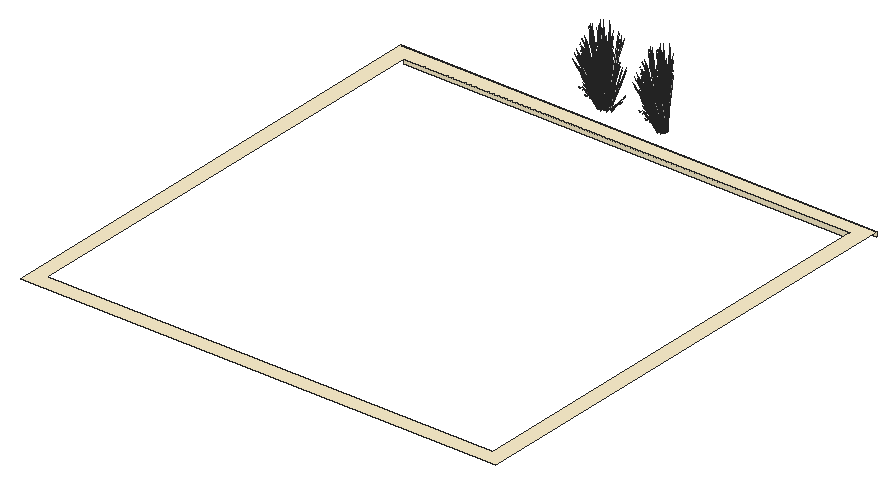
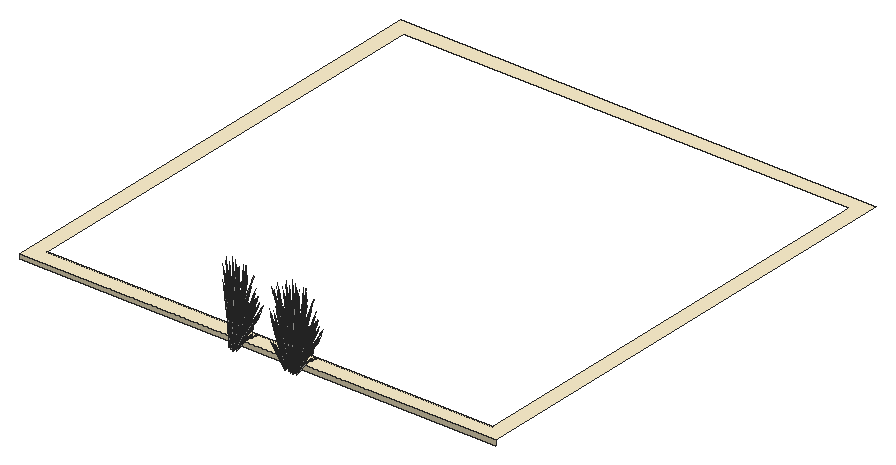
# SketchUp Ruby script. Lengths in inches.
U = 1.inch
M = Sketchup.active_model
def pt(a) = Geom::Point3d.new(a.map { |v| v * U })
def face(e, loops, mat)
  f = e.add_face(loops[0].map { |a| pt(a) })
  loops[1..].each { |l| e.add_face(l.map { |a| pt(a) }).erase! }
  f.material = f.back_material = mat if mat
  f
end
# faces: each face lists its corners as indices into pts; further lists are holes
def faces(e, pts, list, mat = nil) = list.each { |f| face(e, (f[0].is_a?(Array) ? f : [f]).map { |l| l.map { |i| pts[i] } }, mat) }
# xy, xz, yz: faces in a plane at the given z, y or x. An outline is a flat list of corners, or four numbers for a rectangle; further outlines are holes
def ring(l) = l.size == 4 ? [[l[0], l[1]], [l[2], l[1]], [l[2], l[3]], [l[0], l[3]]] : l.each_slice(2).to_a
def flat(e, list, mat, &to3) = list.each { |f| face(e, (f[0].is_a?(Array) ? f : [f]).map { |l| ring(l).map { |u, v| to3.(u, v) } }, mat) }
def xy(e, z, list, mat = nil) = flat(e, list, mat) { |x, y| [x, y, z] }
def xz(e, y, list, mat = nil) = flat(e, list, mat) { |x, z| [x, y, z] }
def yz(e, x, list, mat = nil) = flat(e, list, mat) { |y, z| [x, y, z] }
def lines(e, pts, list) = list.each { |a, b| e.add_line(pt(pts[a]), pt(pts[b])) }
# prism: a flat outline (further loops are holes) pulled along v
def prism(e, loops, v, mat = nil)
  f = face(e, loops, mat); d = Geom::Vector3d.new(v.map { |x| x * U })
  f.pushpull(f.normal.samedirection?(d) ? d.length : -d.length)
end
def box(e, o, s, mat = nil) = prism(e, [[o, [o[0] + s[0], o[1], o[2]], [o[0] + s[0], o[1] + s[1], o[2]], [o[0], o[1] + s[1], o[2]]]], [0, 0, s[2]], mat)
def at(x, y, z, deg = 0) = Geom::Transformation.translation(pt([x, y, z])) * Geom::Transformation.rotation(ORIGIN, Z_AXIS, deg.degrees)
def axes(o, x, y, z) = Geom::Transformation.new([*x, 0, *y, 0, *z, 0, *pt(o).to_a, 1])
def part(name) = M.definitions.add(name)
# library, detail: a bought-in or finely detailed component or shape, given as its bounding box
def library(name, o, s) = part(name).tap { |d| box(d.entities, o, s) }
def detail(e, o, s) = box(e.add_group.entities, o, s)
def put(e, d, t, mat = nil) = e.add_instance(d, t).tap { |i| i.material = mat if mat }
def group(e, t, mat = nil) = e.add_group.tap { |g| g.transformation = t; g.material = mat if mat }.entities
root = M.entities
M.materials.add("D01_Frost_White").color = [255, 242, 206]
M.materials.add("LightPink_Translucent").color = [144, 107, 117]
M.materials["LightPink_Translucent"].alpha = 0.75
c1 = part("blade")
p = [[2.15,0.21,22],[0,0.17,0],[0.09,0.45,0],[2.18,0.31,22],[2.29,0.31,22],[0.38,0.45,0],
  [2.48,0.24,33],[2.49,0.24,33],[2.48,0.22,33]]
faces(c1.entities,p,[[0,1,2,3],[4,5,2,3],[6,3,4,7],[8,0,3,6]])
c2 = part("seeds")
p = [[0.3,-0.1,1.38],[-0.01,-0.03,1.59],[-0.01,-0.03,0.03],[0.14,-0.07,-0.07],[0.29,-0.03,3],[0.15,0.01,3.11]]
faces(c2.entities,p,[[0,1,2,3],[1,0,4,5]],"LightPink_Translucent")
c3 = part("blade with seeds")
put(c3.entities,c1,at(0,0,0))
put(c3.entities,c2,axes([2.4,0.25,30.99],[1.5799,-0.05474,1.17369],[-0.12525,1.92788,0.29478],[-0.07173,-0.02425,1.56792]))
xy(root,2,[[[660.12,282,852,474],[666.12,288,846,468]]],"D01_Frost_White")
xz(root,468,[[666.12,0,846,2]],"D01_Frost_White")
xz(root,474,[[660.12,0,852,2]],"D01_Frost_White")
put(root,c3,axes([735.64,479.97,3.9375],[0.10505,0.10498,0.85688],[-0.48542,0.08838,0.06928],[-0.10971,-0.1648,0.36631]))
put(root,c3,axes([759.85,479.97,3.9375],[0.10505,0.10498,0.85688],[-0.48542,0.08838,0.06928],[-0.10971,-0.1648,0.36631]))
put(root,c3,axes([736.45,479.28,4.36],[-0.07029,-0.04584,0.87472],[-0.46908,0.02906,-0.13834],[-0.07486,-0.10965,0.07015]))
put(root,c3,axes([760.65,479.28,4.36],[-0.07029,-0.04584,0.87472],[-0.46908,0.02906,-0.13834],[-0.07486,-0.10965,0.07015]))
put(root,c3,axes([737.53,479.82,3.3],[-0.13063,0.06618,0.71501],[-0.39122,-0.11583,-0.15377],[0.07252,-0.14406,0.3057]))
put(root,c3,axes([761.74,479.82,3.3],[-0.13063,0.06618,0.71501],[-0.39122,-0.11583,-0.15377],[0.07252,-0.14406,0.3057]))
put(root,c3,axes([736.9375,480.05,4.49],[-0.21934,-0.26585,-0.35523],[0.45151,-0.14816,0.04287],[-0.05129,-0.12845,0.5025]))
put(root,c3,axes([761.14,480.05,4.49],[-0.21934,-0.26585,-0.35523],[0.45151,-0.14816,0.04287],[-0.05129,-0.12845,0.5025]))
put(root,c3,axes([735.51,479.69,3.3],[-0.02783,0.10696,0.71501],[-0.40683,0.08954,-0.15377],[-0.0951,-0.13825,0.3057]))
put(root,c3,axes([759.71,479.69,3.3],[-0.02783,0.10696,0.71501],[-0.40683,0.08954,-0.15377],[-0.0951,-0.13825,0.3057]))
put(root,c3,axes([736.56,479.46,2.75],[-0.07708,0.01178,0.88171],[-0.42627,-0.1326,-0.1347],[0.00715,-0.1106,0.15018]))
put(root,c3,axes([760.76,479.46,2.75],[-0.07708,0.01178,0.88171],[-0.42627,-0.1326,-0.1347],[0.00715,-0.1106,0.15018]))
put(root,c3,axes([737.85,480.31,4.49],[0.01196,-0.30243,-0.35523],[0.50354,0.02031,0.04287],[0.05314,-0.12813,0.5025]))
put(root,c3,axes([762.05,480.31,4.49],[0.01196,-0.30243,-0.35523],[0.50354,0.02031,0.04287],[0.05314,-0.12813,0.5025]))
put(root,c3,axes([738.55,479.84,4.36],[-0.00444,-0.06507,0.87472],[-0.37468,-0.18807,-0.13834],[0.05793,-0.114,0.07015]))
put(root,c3,axes([762.75,479.84,4.36],[-0.00444,-0.06507,0.87472],[-0.37468,-0.18807,-0.13834],[0.05793,-0.114,0.07015]))
put(root,c3,axes([736.98,479.82,4.26],[0.13855,-0.25143,-0.17707],[0.4042,0.07334,0.2286],[-0.03706,-0.10123,0.4374]))
put(root,c3,axes([761.18,479.82,4.26],[0.13855,-0.25143,-0.17707],[0.4042,0.07334,0.2286],[-0.03706,-0.10123,0.4374]))
put(root,c3,axes([737.28,480.16,3.9375],[-0.08557,0.11238,0.85688],[-0.35897,-0.23257,0.06928],[0.16194,-0.14495,0.36631]))
put(root,c3,axes([738.45,479.6,4.35],[-0.04667,0.02497,0.88692],[-0.45726,-0.08426,-0.08381],[-0.01655,-0.10898,0.15695]))
put(root,c3,axes([762.65,479.6,4.35],[-0.04667,0.02497,0.88692],[-0.45726,-0.08426,-0.08381],[-0.01655,-0.10898,0.15695]))
put(root,c3,axes([736.77,480,4.34],[-0.45175,-0.08196,-0.25549],[0.15485,-0.28101,-0.1979],[-0.04142,-0.11314,0.48886]))
put(root,c3,axes([760.97,480,4.34],[-0.45175,-0.08196,-0.25549],[0.15485,-0.28101,-0.1979],[-0.04142,-0.11314,0.48886]))
put(root,c3,axes([737.05,479.29,3.38],[0.05895,0.19066,0.5743],[-0.32704,-0.1056,0.42196],[0.03519,-0.09762,0.12649]))
put(root,c3,axes([761.25,479.29,3.38],[0.05895,0.19066,0.5743],[-0.32704,-0.1056,0.42196],[0.03519,-0.09762,0.12649]))
put(root,c3,axes([737.75,480.21,4.34],[-0.32898,-0.21969,-0.25549],[0.34753,-0.1924,-0.1979],[0.05006,-0.11162,0.48886]))
put(root,c3,axes([761.95,480.21,4.34],[-0.32898,-0.21969,-0.25549],[0.34753,-0.1924,-0.1979],[0.05006,-0.11162,0.48886]))
put(root,c3,axes([735.96,479.125,4.35],[-0.00857,0.03919,0.88692],[-0.42284,0.14223,-0.08381],[-0.12443,-0.0727,0.15695]))
put(root,c3,axes([760.17,479.125,4.35],[-0.00857,0.03919,0.88692],[-0.42284,0.14223,-0.08381],[-0.12443,-0.0727,0.15695]))
put(root,c3,axes([735.87,479.82,4.55],[0.51193,-0.08404,0.26881],[0.08885,0.32966,0.22165],[-0.1204,-0.09716,0.55625]))
put(root,c3,axes([760.07,479.82,4.55],[0.51193,-0.08404,0.26881],[0.08885,0.32966,0.22165],[-0.1204,-0.09716,0.55625]))
put(root,c3,axes([737.03,479.88,4.37],[0.45283,0.08548,0.24001],[-0.15485,0.28101,0.1979],[-0.02721,-0.11051,0.49665]))
put(root,c3,axes([761.23,479.88,4.37],[0.45283,0.08548,0.24001],[-0.15485,0.28101,0.1979],[-0.02721,-0.11051,0.49665]))
put(root,c3,axes([737.16,479.98,4.52],[-0.44971,0.15222,-0.0608],[-0.221,-0.27017,-0.33747],[-0.05933,-0.11385,0.51278]))
put(root,c3,axes([761.36,479.98,4.52],[-0.44971,0.15222,-0.0608],[-0.221,-0.27017,-0.33747],[-0.05933,-0.11385,0.51278]))
put(root,c3,axes([738.09,480.32,4.52],[-0.50507,-0.0162,-0.0608],[0.01381,-0.30672,-0.33747],[0.03508,-0.11813,0.51278]))
put(root,c3,axes([762.3,480.32,4.52],[-0.50507,-0.0162,-0.0608],[0.01381,-0.30672,-0.33747],[0.03508,-0.11813,0.51278]))
put(root,c3,axes([738.06,480.13,4.26],[0.31095,-0.17214,-0.17707],[0.29435,0.19656,0.2286],[0.04479,-0.09987,0.4374]))
put(root,c3,axes([762.26,480.13,4.26],[0.31095,-0.17214,-0.17707],[0.29435,0.19656,0.2286],[0.04479,-0.09987,0.4374]))
put(root,c3,axes([735.37,479.52,3.38],[0.23972,0.1138,0.5743],[-0.34912,0.06841,0.42196],[-0.0747,-0.08746,0.12649]))
put(root,c3,axes([759.57,479.52,3.38],[0.23972,0.1138,0.5743],[-0.34912,0.06841,0.42196],[-0.0747,-0.08746,0.12649]))
put(root,c3,axes([737.15,479.86,4.37],[0.33863,-0.11112,0.03215],[0.16575,0.20263,0.2531],[-0.0327,-0.08932,0.38595]))
put(root,c3,axes([761.35,479.86,4.37],[0.33863,-0.11112,0.03215],[0.16575,0.20263,0.2531],[-0.0327,-0.08932,0.38595]))
put(root,c3,axes([735.95,480.125,4.49],[-0.39186,-0.15803,-0.35523],[0.27849,-0.27693,0.04287],[-0.14198,-0.09436,0.5025]))
put(root,c3,axes([760.15,480.125,4.49],[-0.39186,-0.15803,-0.35523],[0.27849,-0.27693,0.04287],[-0.14198,-0.09436,0.5025]))
put(root,c3,axes([735.8125,479.92,4.26],[-0.07098,-0.26335,-0.17707],[0.40574,-0.06954,0.2286],[-0.10898,-0.07547,0.4374]))
put(root,c3,axes([760.02,479.92,4.26],[-0.07098,-0.26335,-0.17707],[0.40574,-0.06954,0.2286],[-0.10898,-0.07547,0.4374]))
put(root,c3,axes([735.99,479.89,4.37],[0.20887,-0.2077,0.03215],[0.29744,0.12092,0.2531],[-0.09616,-0.06659,0.38595]))
put(root,c3,axes([760.19,479.89,4.37],[0.20887,-0.2077,0.03215],[0.29744,0.12092,0.2531],[-0.09616,-0.06659,0.38595]))
put(root,c3,axes([735.18,479.86,2.75],[-0.04451,0.04307,0.88171],[-0.44986,0.09286,-0.1347],[-0.10868,-0.08448,0.15018]))
put(root,c3,axes([759.38,479.86,2.75],[-0.04451,0.04307,0.88171],[-0.44986,0.09286,-0.1347],[-0.10868,-0.08448,0.15018]))
put(root,c3,axes([735.92,481.05,3.05],[-0.18873,-0.33528,-0.34918],[0.54365,-0.12075,-0.09164],[-0.02086,-0.11353,0.77075]))
put(root,c3,axes([760.125,481.05,3.05],[-0.18873,-0.33528,-0.34918],[0.54365,-0.12075,-0.09164],[-0.02086,-0.11353,0.77075]))
put(root,c3,axes([734.94,480.3,3.9375],[0.1707,0.05633,0.85688],[-0.35326,0.23632,0.06928],[-0.22018,-0.10661,0.36631]))
put(root,c3,axes([759.14,480.3,3.9375],[0.1707,0.05633,0.85688],[-0.35326,0.23632,0.06928],[-0.22018,-0.10661,0.36631]))
put(root,c3,axes([738.45,480.02,2.75],[-0.06878,-0.02576,0.88171],[-0.17668,-0.28776,-0.1347],[0.11919,-0.07809,0.15018]))
put(root,c3,axes([737.02,480.09,4.53],[-0.13855,0.25143,0.17707],[-0.4042,-0.07334,-0.2286],[-0.03706,-0.10123,0.4374]))
put(root,c3,axes([761.23,480.09,4.53],[-0.13855,0.25143,0.17707],[-0.4042,-0.07334,-0.2286],[-0.03706,-0.10123,0.4374]))
put(root,c3,axes([735.77,480.13,4.34],[-0.45348,0.07772,-0.25549],[-0.07933,-0.29434,-0.1979],[-0.1218,-0.08435,0.48886]))
put(root,c3,axes([759.97,480.13,4.34],[-0.45348,0.07772,-0.25549],[-0.07933,-0.29434,-0.1979],[-0.1218,-0.08435,0.48886]))
put(root,c3,axes([738.06,480.19,4.37],[0.32725,0.22308,0.24001],[-0.34753,0.1924,0.1979],[0.06036,-0.10466,0.49665]))
put(root,c3,axes([762.26,480.19,4.37],[0.32725,0.22308,0.24001],[-0.34753,0.1924,0.1979],[0.06036,-0.10466,0.49665]))
put(root,c3,axes([736.08,479.87,4.72],[-0.30671,0.31344,-0.0681],[-0.44417,-0.18058,-0.37797],[-0.1544,-0.08856,0.57432]))
put(root,c3,axes([760.28,479.87,4.72],[-0.30671,0.31344,-0.0681],[-0.44417,-0.18058,-0.37797],[-0.1544,-0.08856,0.57432]))
put(root,c3,axes([738.18,480.22,4.37],[0.37765,0.01523,0.03215],[-0.01035,0.23004,0.2531],[0.03952,-0.08812,0.38595]))
put(root,c3,axes([762.38,480.22,4.37],[0.37765,0.01523,0.03215],[-0.01035,0.23004,0.2531],[0.03952,-0.08812,0.38595]))
put(root,c3,axes([737.9,480.37,4.53],[-0.31095,0.17214,0.17707],[-0.29435,-0.19656,-0.2286],[0.04479,-0.09987,0.4374]))
put(root,c3,axes([762.1,480.37,4.53],[-0.31095,0.17214,0.17707],[-0.29435,-0.19656,-0.2286],[0.04479,-0.09987,0.4374]))
put(root,c3,axes([738.44,480.84,4.49],[0.24005,-0.25798,-0.35523],[0.42065,0.18334,0.04287],[0.14333,-0.09347,0.5025]))
put(root,c3,axes([735.85,480.08,3.1875],[-0.28732,-0.32763,0],[0.4807,-0.18271,-0.25804],[0.10948,-0.04161,0.81856]))
put(root,c3,axes([760.05,480.08,3.1875],[-0.28732,-0.32763,0],[0.4807,-0.18271,-0.25804],[0.10948,-0.04161,0.81856]))
put(root,c3,axes([738.43,480.72,4.34],[-0.11806,-0.29854,-0.25549],[0.44709,-0.05222,-0.1979],[0.12812,-0.08019,0.48886]))
put(root,c3,axes([736.48,479.69,3.0625],[-0.31757,0.18757,-0.01946],[-0.29098,-0.20543,-0.08825],[-0.02049,-0.05821,0.29107]))
put(root,c3,axes([760.68,479.69,3.0625],[-0.31757,0.18757,-0.01946],[-0.29098,-0.20543,-0.08825],[-0.02049,-0.05821,0.29107]))
put(root,c3,axes([734.91,479.78,4.36],[-0.09888,-0.00231,0.87472],[-0.3148,0.23079,-0.13834],[-0.16797,-0.04716,0.07015]))
put(root,c3,axes([759.11,479.78,4.36],[-0.09888,-0.00231,0.87472],[-0.3148,0.23079,-0.13834],[-0.16797,-0.04716,0.07015]))
put(root,c3,axes([738.64,480.93,4.52],[-0.4251,-0.18028,-0.0608],[0.24491,-0.26108,-0.33747],[0.1201,-0.09075,0.51278]))
put(root,c3,axes([736.89,481.91,3.66],[0.39713,0.13184,0.7563],[-0.38905,0.28403,0.29908],[-0.17427,-0.16834,0.63403]))
put(root,c3,axes([761.09,481.91,3.66],[0.39713,0.13184,0.7563],[-0.38905,0.28403,0.29908],[-0.17427,-0.16834,0.63403]))
put(root,c3,axes([736.05,480.13,4.53],[0.07098,0.26335,0.17707],[-0.40574,0.06954,-0.2286],[-0.10898,-0.07547,0.4374]))
put(root,c3,axes([760.26,480.13,4.53],[0.07098,0.26335,0.17707],[-0.40574,0.06954,-0.2286],[-0.10898,-0.07547,0.4374]))
put(root,c3,axes([734.8125,481,3.01],[0,-0.32696,-0.24825],[0.51416,0,0],[0,-0.07447,0.78752]))
put(root,c3,axes([759.01,481,3.01],[0,-0.32696,-0.24825],[0.51416,0,0],[0,-0.07447,0.78752]))
put(root,c3,axes([736.24,480.03,3.01],[0.4301,-0.16348,-0.24825],[0.25708,0.29314,0],[0.09796,-0.03723,0.78752]))
put(root,c3,axes([760.44,480.03,3.01],[0.4301,-0.16348,-0.24825],[0.25708,0.29314,0],[0.09796,-0.03723,0.78752]))
put(root,c3,axes([738.79,480.6,3.3],[-0.16417,-0.00968,0.71501],[-0.16819,-0.25979,-0.15377],[0.20169,-0.07349,0.3057]))
put(root,c3,axes([734.83,480.3,4.55],[0.37952,-0.24129,0.26881],[0.32731,0.25625,0.22165],[-0.17806,-0.04451,0.55625]))
put(root,c3,axes([759.04,480.3,4.55],[0.37952,-0.24129,0.26881],[0.32731,0.25625,0.22165],[-0.17806,-0.04451,0.55625]))
put(root,c3,axes([739.69,480.85,4.35],[-0.06002,-0.00248,0.88692],[-0.24926,-0.26607,-0.08381],[0.1001,-0.08748,0.15695]))
put(root,c3,axes([736.75,480.7,3.03],[0.30954,-0.24575,-0.31177],[0.38452,0.22284,-0.08182],[0.12404,-0.0613,0.68817]))
put(root,c3,axes([760.95,480.7,3.03],[0.30954,-0.24575,-0.31177],[0.38452,0.22284,-0.08182],[0.12404,-0.0613,0.68817]))
put(root,c3,axes([738.98,480.12,3.38],[-0.15307,0.16644,0.5743],[-0.13157,-0.22361,0.42196],[0.12643,-0.05603,0.12649]))
put(root,c3,axes([738.76,480.75,4.26],[0.40003,-0.04673,-0.17707],[0.10563,0.26712,0.2286],[0.11464,-0.07175,0.4374]))
put(root,c3,axes([735.01,480.3,4.37],[0.02314,-0.24862,0.03215],[0.34943,0.00682,0.2531],[-0.13385,-0.02602,0.38595]))
put(root,c3,axes([759.21,480.3,4.37],[0.02314,-0.24862,0.03215],[0.34943,0.00682,0.2531],[-0.13385,-0.02602,0.38595]))
put(root,c3,axes([736.21,481.14,3.11],[0.22297,-0.29461,-0.2237],[0.4633,0.14179,0.10766],[0,-0.06791,0.71822]))
put(root,c3,axes([760.41,481.14,3.11],[0.22297,-0.29461,-0.2237],[0.4633,0.14179,0.10766],[0,-0.06791,0.71822]))
put(root,c3,axes([734.875,480.38,4.26],[-0.26148,-0.20471,-0.17707],[0.29857,-0.19378,0.2286],[-0.1517,-0.02948,0.4374]))
put(root,c3,axes([759.08,480.38,4.26],[-0.26148,-0.20471,-0.17707],[0.29857,-0.19378,0.2286],[-0.1517,-0.02948,0.4374]))
put(root,c3,axes([736.41,480.99,3.33],[-0.05355,-0.37308,-0.14548],[0.55775,-0.02256,-0.25001],[0.09822,-0.04969,0.79854]))
put(root,c3,axes([760.62,480.99,3.33],[-0.05355,-0.37308,-0.14548],[0.55775,-0.02256,-0.25001],[0.09822,-0.04969,0.79854]))
put(root,c3,axes([735.03,481.01,3.01],[0.32079,-0.20399,-0.15489],[0.32079,0.20399,0.15489],[0,-0.06571,0.69487]))
put(root,c3,axes([759.23,481.01,3.01],[0.32079,-0.20399,-0.15489],[0.32079,0.20399,0.15489],[0,-0.06571,0.69487]))
put(root,c3,axes([734.9,480.03,3.0625],[-0.13257,0.26698,-0.01946],[-0.40802,-0.08212,-0.08825],[-0.06195,-0.04367,0.29107]))
put(root,c3,axes([759.1,480.03,3.0625],[-0.13257,0.26698,-0.01946],[-0.40802,-0.08212,-0.08825],[-0.06195,-0.04367,0.29107]))
put(root,c3,axes([738.4375,480.9,4.53],[-0.40003,0.04673,0.17707],[-0.10563,-0.26712,-0.2286],[0.11464,-0.07175,0.4374]))
put(root,c3,axes([736.15,481.38,3.33],[-0.51755,-0.15601,-0.14548],[0.2492,-0.32927,-0.25001],[-0.01626,-0.08084,0.79854]))
put(root,c3,axes([760.36,481.38,3.33],[-0.51755,-0.15601,-0.14548],[0.2492,-0.32927,-0.25001],[-0.01626,-0.08084,0.79854]))
put(root,c3,axes([734.68,481.25,3.1875],[-0.57465,0,0],[0,-0.36542,-0.25804],[0,-0.08323,0.81856]))
put(root,c3,axes([758.88,481.25,3.1875],[-0.57465,0,0],[0,-0.36542,-0.25804],[0,-0.08323,0.81856]))
put(root,c3,axes([734.78,480.6,3.3],[0.08973,0.09103,0.71501],[-0.20675,0.24743,-0.15377],[-0.2123,-0.05914,0.3057]))
put(root,c3,axes([758.98,480.6,3.3],[0.08973,0.09103,0.71501],[-0.20675,0.24743,-0.15377],[-0.2123,-0.05914,0.3057]))
put(root,c3,axes([736.34,480.16,3.01],[0.42874,0.0809,-0.15489],[-0.10795,0.28489,0.15489],[0.08643,-0.03285,0.69487]))
put(root,c3,axes([760.54,480.16,3.01],[0.42874,0.0809,-0.15489],[-0.10795,0.28489,0.15489],[0.08643,-0.03285,0.69487]))
put(root,c3,axes([735.15,480.52,4.49],[-0.45939,-0.00787,-0.35523],[0.03085,-0.3315,0.04287],[-0.19462,-0.03498,0.5025]))
put(root,c3,axes([759.35,480.52,4.49],[-0.45939,-0.00787,-0.35523],[0.03085,-0.3315,0.04287],[-0.19462,-0.03498,0.5025]))
put(root,c3,axes([738.8,480.86,4.37],[0.31549,0.13751,0.03215],[-0.18368,0.19581,0.2531],[0.10115,-0.06331,0.38595]))
put(root,c3,axes([738.71,480.8,4.37],[0.11397,0.30091,0.24001],[-0.44709,0.05222,0.1979],[0.13177,-0.07077,0.49665]))
put(root,c3,axes([739.92,481.17,4.36],[0.06377,-0.0498,0.87472],[-0.08162,-0.30549,-0.13834],[0.16001,-0.05792,0.07015]))
put(root,c3,axes([735.13,481.15,3.17],[-0.42746,0.27488,0.15378],[-0.42772,-0.27199,-0.18246],[-0.01493,-0.07806,0.82443]))
put(root,c3,axes([759.33,481.15,3.17],[-0.42746,0.27488,0.15378],[-0.42772,-0.27199,-0.18246],[-0.01493,-0.07806,0.82443]))
put(root,c3,axes([734.53,479.98,4.35],[0.03407,0.03263,0.88692],[-0.16424,0.29331,-0.08381],[-0.16634,0.00212,0.15695]))
put(root,c3,axes([758.73,479.98,4.35],[0.03407,0.03263,0.88692],[-0.16424,0.29331,-0.08381],[-0.16634,0.00212,0.15695]))
put(root,c3,axes([736.49,481.28,3.22],[0.5178,0.15847,0.12032],[-0.2492,0.32927,0.25001],[0,-0.0759,0.80271]))
put(root,c3,axes([760.6875,481.28,3.22],[0.5178,0.15847,0.12032],[-0.2492,0.32927,0.25001],[0,-0.0759,0.80271]))
put(root,c3,axes([736.29,481.73,3.22],[0.1218,-0.38743,-0.11714],[0.57753,0.06753,0.25635],[-0.10091,-0.0535,0.7822]))
put(root,c3,axes([760.49,481.73,3.22],[0.1218,-0.38743,-0.11714],[0.57753,0.06753,0.25635],[-0.10091,-0.0535,0.7822]))
put(root,c3,axes([735,480.58,4.34],[-0.3337,0.21658,-0.25549],[-0.29224,-0.22879,-0.1979],[-0.16955,-0.03295,0.48886]))
put(root,c3,axes([759.2,480.58,4.34],[-0.3337,0.21658,-0.25549],[-0.29224,-0.22879,-0.1979],[-0.16955,-0.03295,0.48886]))
put(root,c3,axes([735.25,480.49,4.53],[0.26148,0.20471,0.17707],[-0.29857,0.19378,-0.2286],[-0.1517,-0.02948,0.4374]))
put(root,c3,axes([759.45,480.49,4.53],[0.26148,0.20471,0.17707],[-0.29857,0.19378,-0.2286],[-0.1517,-0.02948,0.4374]))
put(root,c3,axes([734.25,480.87,3.38],[0.2934,-0.0234,0.5743],[-0.18611,0.20614,0.42196],[-0.14499,-0.03092,0.12649]))
put(root,c3,axes([758.45,480.87,3.38],[0.2934,-0.0234,0.5743],[-0.18611,0.20614,0.42196],[-0.14499,-0.03092,0.12649]))
put(root,c3,axes([736.32,481.0625,3.36],[-0.49904,0.02018,0.2237],[-0.04513,-0.33504,-0.10766],[0.08934,-0.03396,0.71822]))
put(root,c3,axes([760.52,481.0625,3.36],[-0.49904,0.02018,0.2237],[-0.04513,-0.33504,-0.10766],[0.08934,-0.03396,0.71822]))
put(root,c3,axes([735.17,480.36,4.52],[-0.02461,0.33251,-0.0608],[-0.4659,-0.00909,-0.33747],[-0.17944,-0.0231,0.51278]))
put(root,c3,axes([759.375,480.36,4.52],[-0.02461,0.33251,-0.0608],[-0.4659,-0.00909,-0.33747],[-0.17944,-0.0231,0.51278]))
put(root,c3,axes([735.03,481.31,3.24],[0,0.32696,0.24825],[-0.51416,0,0],[0,-0.07447,0.78752]))
put(root,c3,axes([759.23,481.31,3.24],[0,0.32696,0.24825],[-0.51416,0,0],[0,-0.07447,0.78752]))
put(root,c3,axes([738.66,481.63,4.52],[-0.23123,-0.29606,-0.0608],[0.41039,-0.14549,-0.33747],[0.17294,-0.03906,0.51278]))
put(root,c3,axes([738.64,481.38,4.34],[0.1245,-0.29741,-0.25549],[0.42685,0.10194,-0.1979],[0.17186,-0.02727,0.48886]))
put(root,c3,axes([737.96,480.17,3.1875],[0.28732,-0.32763,0],[0.4807,0.18271,-0.25804],[0.10948,0.04161,0.81856]))
put(root,c3,axes([734.58,480.8125,3.9375],[0.19062,-0.00741,0.85688],[-0.12645,0.32094,0.06928],[-0.27165,-0.01985,0.36631]))
put(root,c3,axes([758.78,480.8125,3.9375],[0.19062,-0.00741,0.85688],[-0.12645,0.32094,0.06928],[-0.27165,-0.01985,0.36631]))
put(root,c3,axes([736.24,481.57,3.11],[-0.27607,-0.27443,-0.2237],[0.41817,-0.19325,0.10766],[-0.08934,-0.03396,0.71822]))
put(root,c3,axes([760.45,481.57,3.11],[-0.27607,-0.27443,-0.2237],[0.41817,-0.19325,0.10766],[-0.08934,-0.03396,0.71822]))
put(root,c3,axes([736.3,481.18,3.18],[0.1998,0.3656,0.22877],[-0.5709,0.12713,0.08977],[0.00698,-0.06718,0.79428]))
put(root,c3,axes([760.5,481.18,3.18],[0.1998,0.3656,0.22877],[-0.5709,0.12713,0.08977],[0.00698,-0.06718,0.79428]))
put(root,c3,axes([739.1,481.46,2.99],[-0.29599,0.03924,0.70792],[-0.04711,-0.31232,0.04052],[0.20731,-0.04727,0.40283]))
put(root,c3,axes([739.64,481.19,3.13],[-0.28491,-0.20907,-0.03244],[0.31204,-0.19157,-0.14708],[0.08842,-0.01349,0.48512]))
put(root,c3,axes([736.2,481.47,3.36],[-0.22297,0.29461,0.2237],[-0.4633,-0.14179,-0.10766],[0,-0.06791,0.71822]))
put(root,c3,axes([760.4,481.47,3.36],[-0.22297,0.29461,0.2237],[-0.4633,-0.14179,-0.10766],[0,-0.06791,0.71822]))
put(root,c3,axes([737.02,481.21,3.1],[0,-0.37831,0],[0.57465,0,0],[0,0,0.89728]))
put(root,c3,axes([761.22,481.21,3.1],[0,-0.37831,0],[0.57465,0,0],[0,0,0.89728]))
put(root,c3,axes([737.72,480.34,3.24],[-0.4301,-0.16348,0.24825],[0.25708,-0.29314,0],[0.09796,0.03723,0.78752]))
put(root,c3,axes([761.92,480.34,3.24],[-0.4301,-0.16348,0.24825],[0.25708,-0.29314,0],[0.09796,0.03723,0.78752]))
put(root,c3,axes([738.56,481.49,4.49],[0.40382,-0.1444,-0.35523],[0.22505,0.29724,0.04287],[0.19512,-0.03377,0.5025]))
put(root,c3,axes([736,481.67,3.03],[-0.47805,-0.0536,-0.31177],[0.10088,-0.33065,-0.08182],[-0.14266,-0.04007,0.68817]))
put(root,c3,axes([760.2,481.67,3.03],[-0.47805,-0.0536,-0.31177],[0.10088,-0.33065,-0.08182],[-0.14266,-0.04007,0.68817]))
put(root,c3,axes([736.75,480.97,3.18],[-0.38104,0.29672,0.22877],[-0.45269,-0.26192,0.08977],[0.09186,-0.02961,0.79428]))
put(root,c3,axes([760.95,480.97,3.18],[-0.38104,0.29672,0.22877],[-0.45269,-0.26192,0.08977],[0.09186,-0.02961,0.79428]))
put(root,c3,axes([737.16,481.51,3.15],[-0.42746,-0.28142,-0.03066],[0.42772,-0.28159,0],[-0.01493,-0.00983,0.87786]))
put(root,c3,axes([761.37,481.51,3.15],[-0.42746,-0.28142,-0.03066],[0.42772,-0.28159,0],[-0.01493,-0.00983,0.87786]))
put(root,c3,axes([736.09,480.49,3.24],[-0.13276,0.32494,0.08821],[-0.4858,-0.09195,0.17543],[0.08392,-0.00158,0.80203]))
put(root,c3,axes([760.29,480.49,3.24],[-0.13276,0.32494,0.08821],[-0.4858,-0.09195,0.17543],[0.08392,-0.00158,0.80203]))
put(root,c3,axes([738.5,481.54,4.53],[-0.38192,-0.09121,0.17707],[0.11139,-0.2661,-0.2286],[0.15377,-0.0244,0.4374]))
put(root,c3,axes([734.5,481.06,4.37],[0.12984,-0.29812,0.24001],[0.42685,0.10194,0.1979],[-0.16786,0.01792,0.49665]))
put(root,c3,axes([758.7,481.06,4.37],[0.12984,-0.29812,0.24001],[0.42685,0.10194,0.1979],[-0.16786,0.01792,0.49665]))
put(root,c3,axes([735.89,480.75,2.8],[-0.45234,0.1309,0.64464],[-0.14398,-0.37559,0.25048],[0.27777,0.00625,0.73321]))
put(root,c3,axes([737.1,480.85,3.31],[0.08866,-0.29179,0.0724],[0.43315,0.05065,-0.20674],[0.07883,0.02996,0.63372]))
put(root,c3,axes([761.3,480.85,3.31],[0.08866,-0.29179,0.0724],[0.43315,0.05065,-0.20674],[0.07883,0.02996,0.63372]))
put(root,c3,axes([734.47,480.98,4.37],[-0.16879,-0.22293,0.03215],[0.30779,-0.10912,0.2531],[-0.13568,0.02153,0.38595]))
put(root,c3,axes([758.67,480.98,4.37],[-0.16879,-0.22293,0.03215],[0.30779,-0.10912,0.2531],[-0.13568,0.02153,0.38595]))
put(root,c3,axes([736.35,481.54,3.18],[0.58084,0.06889,0.22877],[-0.11821,0.38906,0.08977],[-0.08488,-0.03757,0.79428]))
put(root,c3,axes([760.55,481.54,3.18],[0.58084,0.06889,0.22877],[-0.11821,0.38906,0.08977],[-0.08488,-0.03757,0.79428]))
put(root,c3,axes([739.42,481.26,2.75],[-0.02402,-0.04964,0.88171],[0.16658,-0.29036,-0.1347],[0.16804,-0.00418,0.15018]))
put(root,c3,axes([734.46,481.21,2.75],[0.01165,0.05153,0.88171],[-0.23495,0.26909,-0.1347],[-0.16689,-0.01356,0.15018]))
put(root,c3,axes([758.66,481.21,2.75],[0.01165,0.05153,0.88171],[-0.23495,0.26909,-0.1347],[-0.16689,-0.01356,0.15018]))
put(root,c3,axes([736.92,480.92,3.36],[-0.27607,-0.27443,0.2237],[0.41817,-0.19325,-0.10766],[0.08934,0.03396,0.71822]))
put(root,c3,axes([761.12,480.92,3.36],[-0.27607,-0.27443,0.2237],[0.41817,-0.19325,-0.10766],[0.08934,0.03396,0.71822]))
put(root,c3,axes([735.49,482.18,3.01],[-0.10795,-0.28489,-0.15489],[0.42874,-0.0809,0.15489],[-0.08643,-0.03285,0.69487]))
put(root,c3,axes([759.69,482.18,3.01],[-0.10795,-0.28489,-0.15489],[0.42874,-0.0809,0.15489],[-0.08643,-0.03285,0.69487]))
put(root,c3,axes([736.04,482.16,3.24],[0.49383,-0.08678,0.08821],[0.12194,0.32295,0.17543],[-0.04404,-0.04705,0.80203]))
put(root,c3,axes([760.24,482.16,3.24],[0.49383,-0.08678,0.08821],[0.12194,0.32295,0.17543],[-0.04404,-0.04705,0.80203]))
put(root,c3,axes([737.06,480.94,3.33],[0.46399,-0.21707,-0.14548],[0.30855,0.30672,-0.25001],[0.11448,0.03115,0.79854]))
put(root,c3,axes([738.9,481.51,4.26],[0.38192,0.09121,-0.17707],[-0.11139,0.2661,0.2286],[0.15377,-0.0244,0.4374]))
put(root,c3,axes([735.37,482.3,3.01],[-0.4301,-0.16348,-0.24825],[0.25708,-0.29314,0],[-0.09796,-0.03723,0.78752]))
put(root,c3,axes([759.57,482.3,3.01],[-0.4301,-0.16348,-0.24825],[0.25708,-0.29314,0],[-0.09796,-0.03723,0.78752]))
put(root,c3,axes([738.23,480.36,3.01],[0.4301,0.16348,-0.24825],[-0.25708,0.29314,0],[0.09796,0.03723,0.78752]))
put(root,c3,axes([734.41,481.09,4.26],[-0.38192,-0.09121,-0.17707],[0.11139,-0.2661,0.2286],[-0.15377,0.0244,0.4374]))
put(root,c3,axes([758.61,481.09,4.26],[-0.38192,-0.09121,-0.17707],[0.11139,-0.2661,0.2286],[-0.15377,0.0244,0.4374]))
put(root,c3,axes([737.41,481.3,3.1],[0.51416,0,0],[0,0.33849,0],[0,0,0.89203]))
put(root,c3,axes([761.61,481.3,3.1],[0.51416,0,0],[0,0.33849,0],[0,0,0.89203]))
put(root,c3,axes([736.54,481.72,3.33],[-0.46399,0.21707,-0.14548],[-0.30855,-0.30672,-0.25001],[-0.11448,-0.03115,0.79854]))
put(root,c3,axes([760.74,481.72,3.33],[-0.46399,0.21707,-0.14548],[-0.30855,-0.30672,-0.25001],[-0.11448,-0.03115,0.79854]))
